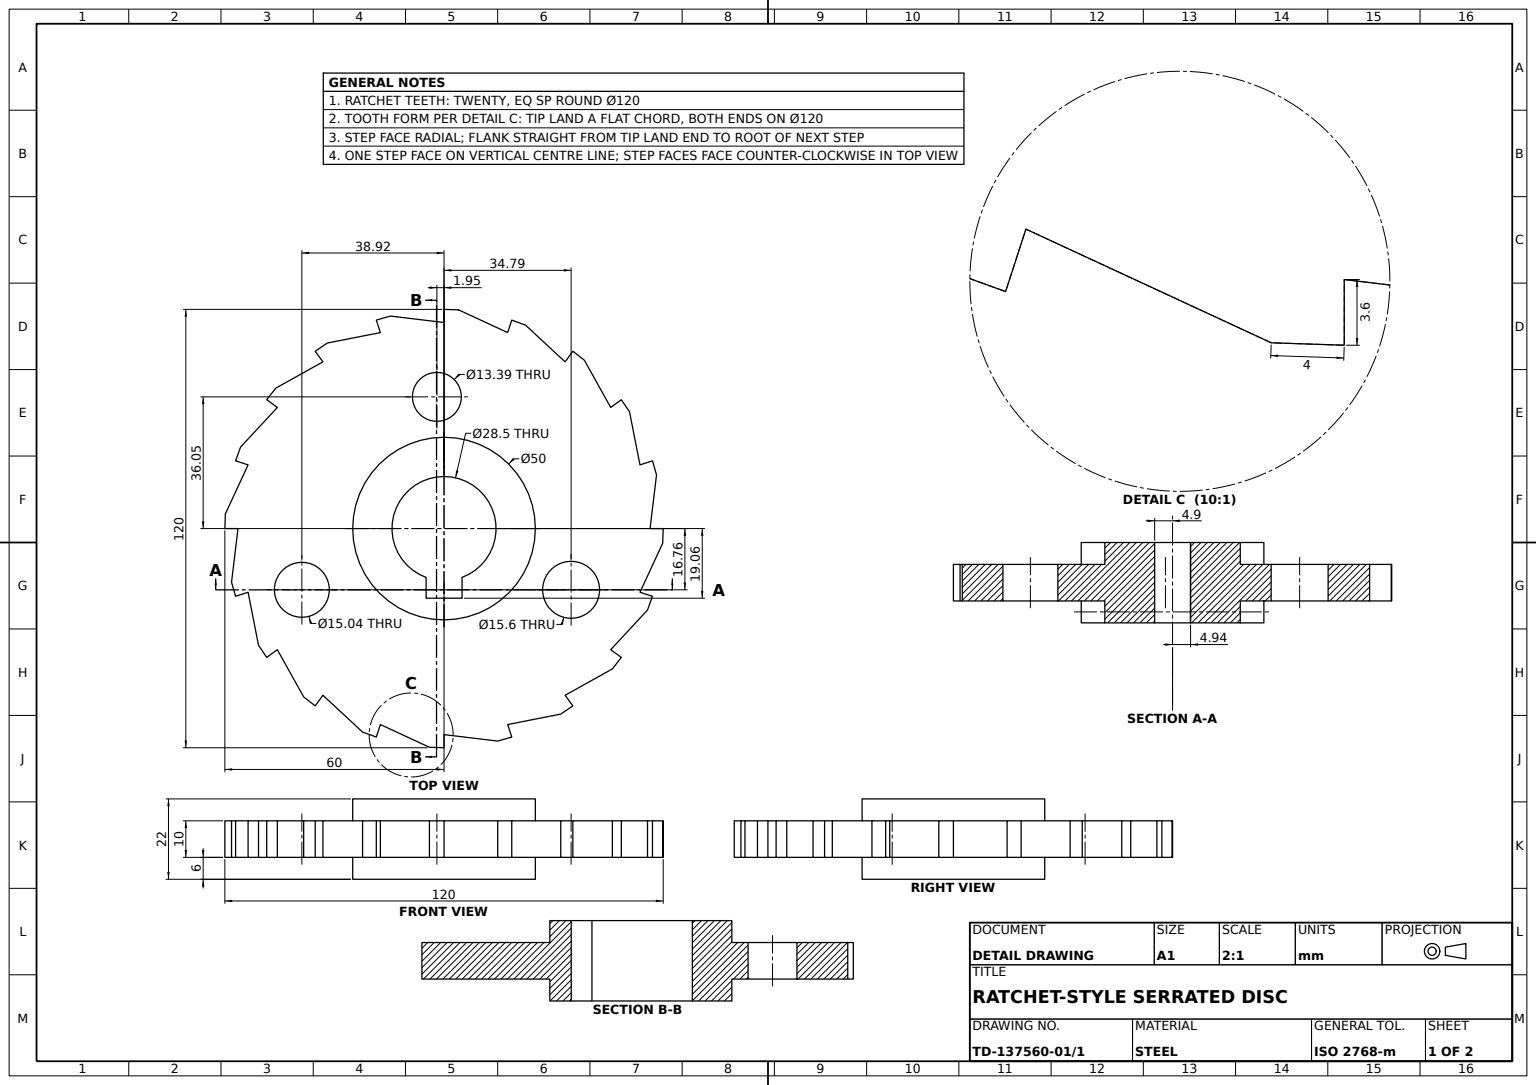
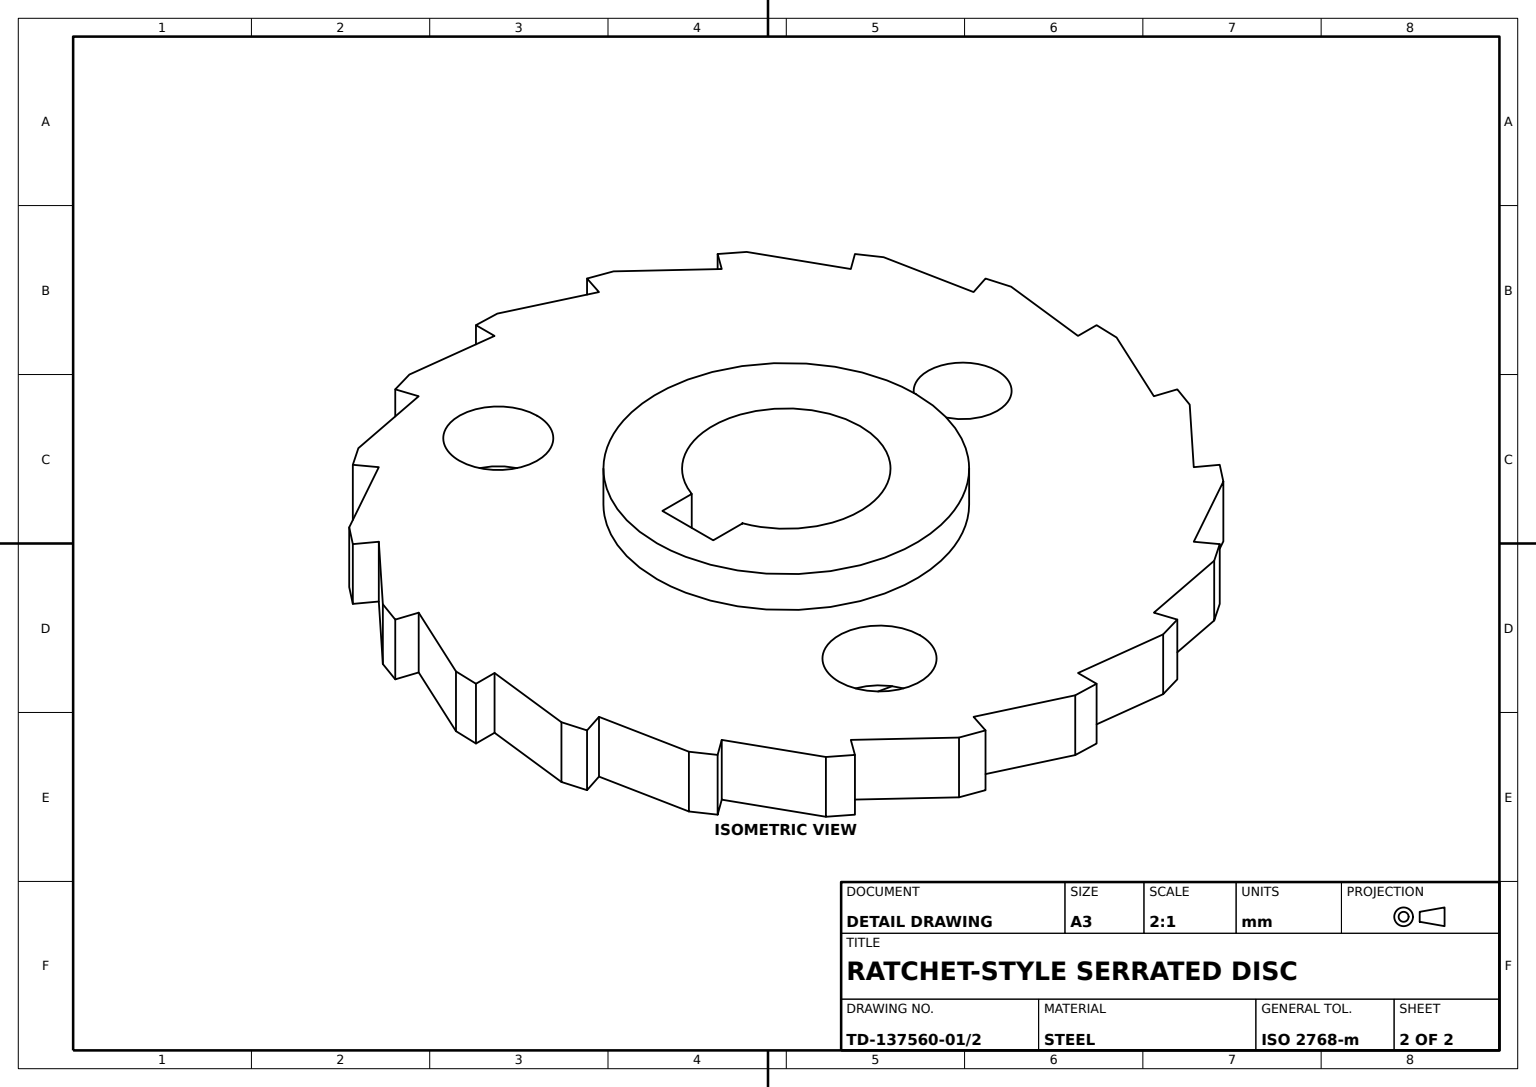
solid
v1 (59.866664,10,-3.997824)
v2 (59.866664,0,-3.997824)
e1 v1 v2 LINE
v3 (53.643191,0,-17.429729)
e2 v2 v3 LINE
v4 (53.643191,10,-17.429729)
e3 v4 v3 LINE
e4 v1 v4 LINE
face PLANE(AX(P(50.810937,10,-23.542486),D(-0.907338164,0,0.420401542),D(0.420401542,0,0.907338164))) rev [e1 e2 -e3 -e4]
v5 (0,10,60)
v6 (0,0,60)
e5 v5 v6 LINE
v7 (3.997824,0,59.866664)
e6 v6 v7 LINE
v8 (3.997824,10,59.866664)
e7 v8 v7 LINE
e8 v5 v8 LINE
face PLANE(AX(P(1.998912,10,59.933332),D(-0.033333726,0,-0.999444277),D(-0.999444277,0,0.033333726))) rev [e5 e6 -e7 -e8]
v9 (-57.063391,0,-18.54102)
v10 (-58.171976,0,-14.69766)
e9 v9 v10 LINE
v11 (-58.171976,10,-14.69766)
e10 v11 v10 LINE
v12 (-57.063391,10,-18.54102)
e11 v12 v11 LINE
e12 v12 v9 LINE
face PLANE(AX(P(-57.617684,10,-16.61934),D(0.96082868,0,0.277143009),D(0.277143009,0,-0.96082868))) rev [e9 -e10 -e11 e12]
v13 (-50.78301,0,-31.954434)
v14 (-53.643191,0,-17.429729)
e13 v13 v14 LINE
v15 (-53.643191,10,-17.429729)
e14 v15 v14 LINE
v16 (-50.78301,10,-31.954434)
e15 v16 v15 LINE
e16 v16 v13 LINE
face PLANE(AX(P(-54.944838,10,-10.819648),D(0.981157821,0,0.193208),D(0.193208,0,-0.981157821))) rev [e13 -e14 -e15 e16]
v17 (-35.267115,10,-48.54102)
v18 (-35.267115,0,-48.54102)
e17 v17 v18 LINE
v19 (-38.42305,0,-46.083286)
e18 v18 v19 LINE
v20 (-38.42305,10,-46.083286)
e19 v20 v19 LINE
e20 v17 v20 LINE
face PLANE(AX(P(-36.845082,10,-47.312153),D(0.614426157,0,0.788974333),D(0.788974333,0,-0.614426157))) rev [e17 e18 -e19 -e20]
v21 (-48.54102,10,35.267115)
v22 (-48.54102,0,35.267115)
e21 v21 v22 LINE
v23 (-45.631624,10,33.153316)
e22 v23 v21 LINE
v24 (-45.631624,0,33.153316)
e23 v23 v24 LINE
e24 v24 v22 LINE
face PLANE(AX(P(0,10,0),D(0.587785252,0,0.809016994),D(0.809016994,0,-0.587785252))) rev [-e21 -e22 e23 e24]
v25 (50.78301,10,31.954434)
v26 (50.78301,0,31.954434)
e25 v25 v26 LINE
v27 (48.54102,10,35.267115)
e26 v27 v25 LINE
v28 (48.54102,0,35.267115)
e27 v27 v28 LINE
e28 v28 v26 LINE
face PLANE(AX(P(49.662015,10,33.610775),D(-0.828160477,0,-0.560491056),D(-0.560491056,0,0.828160477))) rev [-e25 -e26 e27 e28]
v29 (58.171976,0,14.69766)
v30 (56.403789,0,0)
e29 v29 v30 LINE
v31 (56.403789,10,0)
e30 v31 v30 LINE
v32 (58.171976,10,14.69766)
e31 v32 v31 LINE
e32 v32 v29 LINE
face PLANE(AX(P(55.599101,10,-6.688792),D(-0.992841094,0,0.119442714),D(0.119442714,0,0.992841094))) rev [e29 -e30 -e31 e32]
v33 (55.701185,10,-22.301973)
v34 (45.631624,10,-33.153316)
e33 v33 v34 LINE
v35 (55.701185,0,-22.301973)
e34 v33 v35 LINE
v36 (45.631624,0,-33.153316)
e35 v35 v36 LINE
e36 v34 v36 LINE
face PLANE(AX(P(41.049045,10,-38.091678),D(-0.733018652,0,0.680208538),D(0.680208538,0,0.733018652))) rev [-e33 e34 e35 -e36]
v37 (-33.153316,10,-45.631624)
e37 v37 v17 LINE
v38 (-33.153316,0,-45.631624)
e38 v37 v38 LINE
e39 v38 v18 LINE
face PLANE(AX(P(0,10,0),D(-0.809016994,0,0.587785252),D(0.587785252,0,0.809016994))) rev [-e37 e38 e39 -e17]
v39 (18.54102,10,-57.063391)
v40 (18.54102,0,-57.063391)
e40 v39 v40 LINE
v41 (14.69766,0,-58.171976)
e41 v40 v41 LINE
v42 (14.69766,10,-58.171976)
e42 v42 v41 LINE
e43 v39 v42 LINE
face PLANE(AX(P(16.61934,10,-57.617684),D(-0.277143009,0,0.96082868),D(0.96082868,0,0.277143009))) rev [e40 e41 -e42 -e43]
v43 (-33.153316,10,45.631624)
v44 (-33.153316,0,45.631624)
e44 v43 v44 LINE
v45 (-35.267115,0,48.54102)
e45 v44 v45 LINE
v46 (-35.267115,10,48.54102)
e46 v46 v45 LINE
e47 v43 v46 LINE
face PLANE(AX(P(0,10,0),D(0.809016994,0,0.587785252),D(0.587785252,0,-0.809016994))) rev [e44 e45 -e46 -e47]
v47 (-59.866664,0,3.997824)
v48 (-53.643191,0,17.429729)
e48 v47 v48 LINE
v49 (-53.643191,10,17.429729)
e49 v49 v48 LINE
v50 (-59.866664,10,3.997824)
e50 v50 v49 LINE
e51 v50 v47 LINE
face PLANE(AX(P(-50.810937,10,23.542486),D(0.907338164,0,-0.420401542),D(-0.420401542,0,-0.907338164))) rev [e48 -e49 -e50 e51]
v51 (-4.898607,-6,-13.38156)
v52 (-4.898607,16,-13.38156)
e52 v51 v52 LINE
v53 (0,16,14.25)
e53 v52 v53 CIRCLE(AX(P(0,16,0),D(0,1,0),D(0,0,1)),14.25)
v54 (0,-6,14.25)
e54 v54 v53 LINE
e55 v51 v54 CIRCLE(AX(P(0,-6,0),D(0,1,0),D(0,0,1)),14.25)
face CYL(AX(P(0,-41,0),D(0,1,0),D(0,0,1)),14.25) rev [e52 e53 -e54 -e55]
v55 (57.063391,10,18.54102)
v56 (57.063391,0,18.54102)
e56 v55 v56 LINE
e57 v56 v29 LINE
e58 v55 v32 LINE
face PLANE(AX(P(57.617684,10,16.61934),D(-0.96082868,0,-0.277143009),D(-0.277143009,0,0.96082868))) rev [e56 e57 -e32 -e58]
v57 (0,16,25)
v58 (0,16,-25)
e59 v57 v58 CIRCLE(AX(P(0,16,0),D(0,1,0),D(0,0,1)),25)
e60 v58 v57 CIRCLE(AX(P(0,16,0),D(0,1,0),D(0,0,1)),25)
v59 (4.937063,16,-19.059359)
v60 (-4.898607,16,-19.059359)
e61 v59 v60 LINE
v61 (4.937063,16,-13.38156)
e62 v61 v59 LINE
v62 (4.898607,16,-13.38156)
e63 v62 v61 LINE
e64 v53 v62 CIRCLE(AX(P(0,16,0),D(0,1,0),D(0,0,1)),14.25)
e65 v60 v52 LINE
face PLANE(AX(P(0,16,0),D(0,1,0),D(0,0,1))) [e59 e60] [-e61 -e62 -e63 -e64 -e53 -e65]
v63 (-17.429729,10,-53.643191)
v64 (-17.429729,0,-53.643191)
e66 v63 v64 LINE
v65 (-18.54102,0,-57.063391)
e67 v64 v65 LINE
v66 (-18.54102,10,-57.063391)
e68 v66 v65 LINE
e69 v63 v66 LINE
face PLANE(AX(P(0,10,0),D(-0.951056516,0,0.309016994),D(0.309016994,0,0.951056516))) rev [e66 e67 -e68 -e69]
v67 (-17.429729,10,53.643191)
v68 (-17.429729,0,53.643191)
e70 v67 v68 LINE
v69 (-18.54102,0,57.063391)
e71 v68 v69 LINE
v70 (-18.54102,10,57.063391)
e72 v70 v69 LINE
e73 v67 v70 LINE
face PLANE(AX(P(0,10,0),D(0.951056516,0,0.309016994),D(0.309016994,0,-0.951056516))) rev [e70 e71 -e72 -e73]
v71 (17.429729,10,-53.643191)
e74 v71 v39 LINE
v72 (17.429729,0,-53.643191)
e75 v71 v72 LINE
e76 v72 v40 LINE
face PLANE(AX(P(0,10,0),D(-0.951056516,0,-0.309016994),D(-0.309016994,0,0.951056516))) rev [-e40 -e74 e75 e76]
v73 (48.54102,10,-35.267115)
e77 v34 v73 LINE
v74 (48.54102,0,-35.267115)
e78 v36 v74 LINE
e79 v73 v74 LINE
face PLANE(AX(P(0,10,0),D(-0.587785252,0,-0.809016994),D(-0.809016994,0,0.587785252))) rev [-e77 e36 e78 -e79]
v75 (-56.403789,10,0)
v76 (-56.403789,0,0)
e80 v75 v76 LINE
v77 (-60,0,0)
e81 v76 v77 LINE
v78 (-60,10,0)
e82 v78 v77 LINE
e83 v75 v78 LINE
face PLANE(AX(P(0,10,0),D(0,0,1),D(1,0,0))) rev [e80 e81 -e82 -e83]
v79 (-57.063391,0,18.54102)
e84 v48 v79 LINE
v80 (-57.063391,10,18.54102)
e85 v80 v79 LINE
e86 v49 v80 LINE
face PLANE(AX(P(0,10,0),D(0.309016994,0,0.951056516),D(0.951056516,0,-0.309016994))) rev [e49 e84 -e85 -e86]
v81 (33.153316,0,-45.631624)
v82 (35.267115,0,-48.54102)
e87 v81 v82 LINE
v83 (35.267115,10,-48.54102)
e88 v83 v82 LINE
v84 (33.153316,10,-45.631624)
e89 v84 v83 LINE
e90 v84 v81 LINE
face PLANE(AX(P(0,10,0),D(-0.809016994,0,-0.587785252),D(-0.587785252,0,0.809016994))) rev [e87 -e88 -e89 e90]
v85 (0,-6,25)
v86 (0,0,25)
e91 v85 v86 LINE
v87 (0,-6,-25)
e92 v85 v87 CIRCLE(AX(P(0,-6,0),D(0,1,0),D(0,0,1)),25)
v88 (0,0,-25)
e93 v87 v88 LINE
e94 v86 v88 CIRCLE(AX(P(0,0,0),D(0,1,0),D(0,0,1)),25)
face CYL(AX(P(0,-6,0),D(0,1,0),D(0,0,1)),25) [-e91 e92 e93 -e94]
v89 (18.54102,0,57.063391)
v90 (22.301973,0,55.701185)
e95 v89 v90 LINE
v91 (22.301973,10,55.701185)
e96 v91 v90 LINE
v92 (18.54102,10,57.063391)
e97 v92 v91 LINE
e98 v92 v89 LINE
face PLANE(AX(P(20.421496,10,56.382288),D(-0.340547524,0,-0.940227305),D(-0.940227305,0,0.340547524))) rev [e95 -e96 -e97 e98]
v93 (-3.997824,10,-59.866664)
e99 v93 v63 LINE
v94 (-3.997824,0,-59.866664)
e100 v93 v94 LINE
e101 v94 v64 LINE
face PLANE(AX(P(-23.542486,10,-50.810937),D(0.420401542,0,0.907338164),D(0.907338164,0,-0.420401542))) rev [-e99 e100 e101 -e66]
e102 v10 v76 LINE
e103 v14 v9 LINE
v95 (-48.54102,0,-35.267115)
e104 v95 v13 LINE
v96 (-45.631624,0,-33.153316)
e105 v96 v95 LINE
e106 v19 v96 LINE
v97 (-22.301973,0,-55.701185)
e107 v97 v38 LINE
e108 v65 v97 LINE
v98 (0,0,-60)
e109 v98 v94 LINE
v99 (0,0,-56.403789)
e110 v99 v98 LINE
e111 v41 v99 LINE
v100 (31.954434,0,-50.78301)
e112 v100 v72 LINE
e113 v82 v100 LINE
v101 (46.083286,0,-38.42305)
e114 v101 v81 LINE
e115 v74 v101 LINE
v102 (57.063391,0,-18.54102)
e116 v102 v35 LINE
e117 v3 v102 LINE
v103 (60,0,0)
e118 v103 v2 LINE
e119 v30 v103 LINE
v104 (53.643191,0,17.429729)
e120 v104 v56 LINE
e121 v26 v104 LINE
v105 (45.631624,0,33.153316)
e122 v105 v28 LINE
v106 (38.42305,0,46.083286)
e123 v106 v105 LINE
v107 (35.267115,0,48.54102)
e124 v107 v106 LINE
v108 (33.153316,0,45.631624)
e125 v108 v107 LINE
e126 v90 v108 LINE
v109 (17.429729,0,53.643191)
e127 v109 v89 LINE
e128 v7 v109 LINE
v110 (0,0,56.403789)
e129 v110 v6 LINE
v111 (-14.69766,0,58.171976)
e130 v111 v110 LINE
e131 v69 v111 LINE
v112 (-31.954434,0,50.78301)
e132 v112 v68 LINE
e133 v45 v112 LINE
v113 (-46.083286,0,38.42305)
e134 v113 v44 LINE
e135 v22 v113 LINE
v114 (-55.701185,0,22.301973)
e136 v114 v24 LINE
e137 v79 v114 LINE
e138 v77 v47 LINE
v115 (34.789071,0,-24.563742)
v116 (34.789071,0,-8.962359)
e139 v115 v116 CIRCLE(AX(P(34.789071,0,-16.763051),D(0,-1,0),D(0,0,1)),7.800692)
e140 v116 v115 CIRCLE(AX(P(34.789071,0,-16.763051),D(0,-1,0),D(0,0,1)),7.800692)
v117 (-38.922426,0,-24.284994)
v118 (-38.922426,0,-9.241107)
e141 v117 v118 CIRCLE(AX(P(-38.922426,0,-16.763051),D(0,-1,0),D(0,0,1)),7.521943)
e142 v118 v117 CIRCLE(AX(P(-38.922426,0,-16.763051),D(0,-1,0),D(0,0,1)),7.521943)
e143 v88 v86 CIRCLE(AX(P(0,0,0),D(0,1,0),D(0,0,1)),25)
v119 (-1.951862,0,42.746873)
v120 (-1.951862,0,29.357209)
e144 v119 v120 CIRCLE(AX(P(-1.951862,0,36.052041),D(0,-1,0),D(0,0,1)),6.694832)
e145 v120 v119 CIRCLE(AX(P(-1.951862,0,36.052041),D(0,-1,0),D(0,0,1)),6.694832)
face PLANE(AX(P(0,0,0),D(0,1,0),D(0,0,1))) rev [-e102 -e9 -e103 -e13 -e104 -e105 -e106 -e18 -e39 -e107 -e108 -e67 -e101 -e109 -e110 -e111 -e41 -e76 -e112 -e113 -e87 -e114 -e115 -e78 -e35 -e116 -e117 -e2 -e118 -e119 -e29 -e57 -e120 -e121 -e28 -e122 -e123 -e124 -e125 -e126 -e95 -e127 -e128 -e6 -e129 -e130 -e131 -e71 -e132 -e133 -e45 -e134 -e135 -e24 -e136 -e137 -e84 -e48 -e138 -e81] [-e139 -e140] [-e141 -e142] [e94 e143] [-e144 -e145]
e146 v87 v85 CIRCLE(AX(P(0,-6,0),D(0,1,0),D(0,0,1)),25)
face CYL(AX(P(0,-6,0),D(0,1,0),D(0,0,1)),25) [-e143 -e93 e146 e91]
v121 (0,10,56.403789)
e147 v121 v110 LINE
v122 (-14.69766,10,58.171976)
e148 v122 v121 LINE
e149 v122 v111 LINE
face PLANE(AX(P(6.688792,10,55.599101),D(-0.119442714,0,-0.992841094),D(-0.992841094,0,0.119442714))) rev [e130 -e147 -e148 e149]
v123 (-46.083286,10,38.42305)
e150 v123 v113 LINE
e151 v21 v123 LINE
face PLANE(AX(P(-47.312153,10,36.845082),D(0.788974333,0,-0.614426157),D(-0.614426157,0,-0.788974333))) rev [-e150 -e151 e21 e135]
v124 (0,10,-56.403789)
e152 v42 v124 LINE
e153 v124 v99 LINE
face PLANE(AX(P(-6.688792,10,-55.599101),D(0.119442714,0,0.992841094),D(0.992841094,0,-0.119442714))) rev [-e152 e42 e111 -e153]
v125 (57.063391,10,-18.54102)
e154 v125 v33 LINE
e155 v125 v102 LINE
face PLANE(AX(P(56.382288,10,-20.421496),D(-0.940227305,0,0.340547524),D(0.340547524,0,0.940227305))) rev [-e154 e155 e116 -e34]
v126 (60,10,0)
e156 v126 v1 LINE
e157 v126 v103 LINE
face PLANE(AX(P(59.933332,10,-1.998912),D(-0.999444277,0,0.033333726),D(0.033333726,0,0.999444277))) rev [e118 -e1 -e156 e157]
v127 (31.954434,10,-50.78301)
e158 v127 v71 LINE
e159 v127 v100 LINE
face PLANE(AX(P(10.819648,10,-54.944838),D(-0.193208,0,0.981157821),D(0.981157821,0,0.193208))) rev [-e75 -e158 e159 e112]
v128 (34.789071,10,-24.563742)
v129 (34.789071,10,-8.962359)
e160 v128 v129 CIRCLE(AX(P(34.789071,10,-16.763051),D(0,-1,0),D(0,0,1)),7.800692)
e161 v128 v115 LINE
e162 v129 v116 LINE
face CYL(AX(P(34.789071,57,-16.763051),D(0,-1,0),D(0,0,-1)),7.800692) rev [-e160 e161 e139 -e162]
v130 (-55.701185,10,22.301973)
e163 v130 v23 LINE
e164 v130 v114 LINE
face PLANE(AX(P(-41.049045,10,38.091678),D(0.733018652,0,-0.680208538),D(-0.680208538,0,-0.733018652))) rev [e136 -e23 -e163 e164]
v131 (-1.951862,10,42.746873)
e165 v131 v119 LINE
v132 (-1.951862,10,29.357209)
e166 v132 v131 CIRCLE(AX(P(-1.951862,10,36.052041),D(0,-1,0),D(0,0,1)),6.694832)
e167 v132 v120 LINE
face CYL(AX(P(-1.951862,57,36.052041),D(0,-1,0),D(0,0,-1)),6.694832) rev [-e165 -e166 e167 e145]
v133 (46.083286,10,-38.42305)
e168 v133 v84 LINE
e169 v133 v101 LINE
face PLANE(AX(P(27.268985,10,-48.912191),D(-0.486946168,0,0.873431983),D(0.873431983,0,0.486946168))) rev [-e168 e169 e114 -e90]
e170 v11 v75 LINE
face PLANE(AX(P(-55.599101,10,6.688792),D(0.992841094,0,-0.119442714),D(-0.119442714,0,-0.992841094))) rev [e102 -e80 -e170 e10]
v134 (45.631624,10,33.153316)
e171 v134 v27 LINE
e172 v134 v105 LINE
face PLANE(AX(P(0,10,0),D(0.587785252,0,-0.809016994),D(-0.809016994,0,-0.587785252))) rev [-e27 -e171 e172 e122]
v135 (4.937063,-6,-13.38156)
v136 (4.937063,-6,-19.059359)
e173 v135 v136 LINE
e174 v135 v61 LINE
e175 v136 v59 LINE
face PLANE(AX(P(4.937063,-41,-13.38156),D(1,0,0),D(0,0,-1))) rev [-e173 e174 e62 -e175]
e176 v123 v43 LINE
face PLANE(AX(P(-27.268985,10,48.912191),D(0.486946168,0,-0.873431983),D(-0.873431983,0,-0.486946168))) rev [e150 e134 -e44 -e176]
v137 (53.643191,10,17.429729)
e177 v137 v104 LINE
e178 v25 v137 LINE
face PLANE(AX(P(54.944838,10,10.819648),D(-0.981157821,0,-0.193208),D(-0.193208,0,0.981157821))) rev [e121 -e177 -e178 e25]
v138 (-22.301973,10,-55.701185)
e179 v138 v97 LINE
e180 v138 v37 LINE
face PLANE(AX(P(-38.091678,10,-41.049045),D(0.680208538,0,0.733018652),D(0.733018652,0,-0.680208538))) rev [e179 e107 -e38 -e180]
v139 (38.42305,10,46.083286)
e181 v139 v106 LINE
e182 v139 v134 LINE
face PLANE(AX(P(48.912191,10,27.268985),D(-0.873431983,0,-0.486946168),D(-0.486946168,0,0.873431983))) rev [e181 e123 -e172 -e182]
v140 (-38.922426,10,-24.284994)
e183 v140 v117 LINE
v141 (-38.922426,10,-9.241107)
e184 v141 v118 LINE
e185 v140 v141 CIRCLE(AX(P(-38.922426,10,-16.763051),D(0,-1,0),D(0,0,1)),7.521943)
face CYL(AX(P(-38.922426,57,-16.763051),D(0,-1,0),D(0,0,-1)),7.521943) rev [e183 e141 -e184 -e185]
e186 v15 v12 LINE
face PLANE(AX(P(0,10,0),D(-0.309016994,0,0.951056516),D(0.951056516,0,0.309016994))) rev [e103 -e12 -e186 e14]
v142 (-48.54102,10,-35.267115)
e187 v142 v95 LINE
e188 v142 v16 LINE
face PLANE(AX(P(-49.662015,10,-33.610775),D(0.828160477,0,0.560491056),D(0.560491056,0,-0.828160477))) rev [e187 e104 -e16 -e188]
e189 v131 v132 CIRCLE(AX(P(-1.951862,10,36.052041),D(0,-1,0),D(0,0,1)),6.694832)
face CYL(AX(P(-1.951862,57,36.052041),D(0,-1,0),D(0,0,-1)),6.694832) rev [-e167 -e189 e165 e144]
e190 v80 v130 LINE
face PLANE(AX(P(-56.382288,10,20.421496),D(0.940227305,0,-0.340547524),D(-0.340547524,0,-0.940227305))) rev [-e190 e85 e137 -e164]
e191 v31 v126 LINE
face PLANE(AX(P(0,10,0),D(0,0,-1),D(-1,0,0))) rev [-e191 e30 e119 -e157]
e192 v129 v128 CIRCLE(AX(P(34.789071,10,-16.763051),D(0,-1,0),D(0,0,1)),7.800692)
face CYL(AX(P(34.789071,57,-16.763051),D(0,-1,0),D(0,0,-1)),7.800692) rev [-e192 e162 e140 -e161]
v143 (33.153316,10,45.631624)
e193 v91 v143 LINE
e194 v143 v108 LINE
face PLANE(AX(P(38.091678,10,41.049045),D(-0.680208538,0,-0.733018652),D(-0.733018652,0,0.680208538))) rev [-e193 e96 e126 -e194]
v144 (-4.898607,-6,-19.059359)
e195 v144 v51 LINE
v145 (4.898607,-6,-13.38156)
e196 v54 v145 CIRCLE(AX(P(0,-6,0),D(0,1,0),D(0,0,1)),14.25)
e197 v145 v135 LINE
e198 v136 v144 LINE
face PLANE(AX(P(0,-6,0),D(0,1,0),D(0,0,1))) rev [e195 e55 e196 e197 e173 e198] [-e92 -e146]
v146 (0,10,-60)
e199 v146 v93 LINE
e200 v146 v98 LINE
face PLANE(AX(P(-1.998912,10,-59.933332),D(0.033333726,0,0.999444277),D(0.999444277,0,-0.033333726))) rev [e109 -e100 -e199 e200]
v147 (-45.631624,10,-33.153316)
e201 v147 v96 LINE
e202 v20 v147 LINE
face PLANE(AX(P(-48.912191,10,-27.268985),D(0.873431983,0,0.486946168),D(0.486946168,0,-0.873431983))) rev [e19 e106 -e201 -e202]
e203 v141 v140 CIRCLE(AX(P(-38.922426,10,-16.763051),D(0,-1,0),D(0,0,1)),7.521943)
face CYL(AX(P(-38.922426,57,-16.763051),D(0,-1,0),D(0,0,-1)),7.521943) rev [e184 e142 -e183 -e203]
v148 (0,10,-25)
e204 v148 v58 LINE
v149 (0,10,25)
e205 v148 v149 CIRCLE(AX(P(0,10,0),D(0,1,0),D(0,0,1)),25)
e206 v149 v57 LINE
face CYL(AX(P(0,-6,0),D(0,1,0),D(0,0,1)),25) [-e60 -e204 e205 e206]
e207 v121 v5 LINE
face PLANE(AX(P(0,10,0),D(1,0,0),D(0,0,-1))) rev [-e5 -e207 e147 e129]
e208 v83 v127 LINE
face PLANE(AX(P(33.610775,10,-49.662015),D(-0.560491056,0,0.828160477),D(0.828160477,0,0.560491056))) rev [-e159 -e208 e88 e113]
e209 v149 v148 CIRCLE(AX(P(0,10,0),D(0,1,0),D(0,0,1)),25)
v150 (-31.954434,10,50.78301)
e210 v46 v150 LINE
e211 v150 v67 LINE
e212 v70 v122 LINE
v151 (17.429729,10,53.643191)
e213 v8 v151 LINE
e214 v151 v92 LINE
v152 (35.267115,10,48.54102)
e215 v143 v152 LINE
e216 v152 v139 LINE
e217 v137 v55 LINE
e218 v4 v125 LINE
e219 v73 v133 LINE
e220 v124 v146 LINE
e221 v66 v138 LINE
e222 v147 v142 LINE
e223 v78 v50 LINE
face PLANE(AX(P(0,10,0),D(0,1,0),D(0,0,1))) [-e209 -e205] [e151 e176 e47 e210 e211 e73 e212 e148 e207 e8 e213 e214 e97 e193 e215 e216 e182 e171 e26 e178 e217 e58 e31 e191 e156 e4 e218 e154 e33 e77 e219 e168 e89 e208 e158 e74 e43 e152 e220 e199 e99 e69 e221 e180 e37 e20 e202 e222 e188 e15 e186 e11 e170 e83 e223 e50 e86 e190 e163 e22] [e160 e192] [e166 e189] [e185 e203]
face PLANE(AX(P(0,10,0),D(-0.587785252,0,0.809016994),D(0.809016994,0,0.587785252))) rev [-e222 e201 e105 -e187]
face PLANE(AX(P(-20.421496,10,-56.382288),D(0.340547524,0,0.940227305),D(0.940227305,0,-0.340547524))) rev [-e221 e68 e108 -e179]
face PLANE(AX(P(0,10,0),D(0.309016994,0,-0.951056516),D(-0.951056516,0,-0.309016994))) rev [e120 -e56 -e217 e177]
e224 v151 v109 LINE
face PLANE(AX(P(0,10,0),D(0.951056516,0,-0.309016994),D(-0.309016994,0,-0.951056516))) rev [-e214 e224 e127 -e98]
e225 v152 v107 LINE
face PLANE(AX(P(36.845082,10,47.312153),D(-0.614426157,0,-0.788974333),D(-0.788974333,0,0.614426157))) rev [e124 -e181 -e216 e225]
face PLANE(AX(P(47.312153,10,-36.845082),D(-0.788974333,0,0.614426157),D(0.614426157,0,0.788974333))) rev [e79 e115 -e169 -e219]
face PLANE(AX(P(-59.933332,10,1.998912),D(0.999444277,0,-0.033333726),D(-0.033333726,0,-0.999444277))) rev [e82 e138 -e51 -e223]
e226 v145 v62 LINE
face PLANE(AX(P(4.898607,-41,-13.38156),D(0,0,1),D(1,0,0))) rev [-e174 -e197 e226 e63]
face PLANE(AX(P(-16.61934,10,57.617684),D(0.277143009,0,-0.96082868),D(-0.96082868,0,-0.277143009))) rev [e131 -e149 -e212 e72]
face PLANE(AX(P(0,10,0),D(-1,0,0),D(0,0,1))) rev [e153 e110 -e200 -e220]
face PLANE(AX(P(23.542486,10,50.810937),D(-0.420401542,0,-0.907338164),D(-0.907338164,0,0.420401542))) rev [-e224 -e213 e7 e128]
face PLANE(AX(P(0,10,0),D(-0.309016994,0,-0.951056516),D(-0.951056516,0,0.309016994))) rev [e117 -e155 -e218 e3]
e227 v150 v112 LINE
face PLANE(AX(P(-33.610775,10,49.662015),D(0.560491056,0,-0.828160477),D(-0.828160477,0,-0.560491056))) rev [-e227 -e210 e46 e133]
face CYL(AX(P(0,-6,0),D(0,1,0),D(0,0,1)),25) [e209 e204 -e59 -e206]
face PLANE(AX(P(0,10,0),D(0.809016994,0,-0.587785252),D(-0.587785252,0,-0.809016994))) rev [e125 -e225 -e215 e194]
e228 v144 v60 LINE
face PLANE(AX(P(-4.898607,-41,-19.059359),D(0,0,-1),D(-1,0,0))) rev [-e228 -e198 e175 e61]
face PLANE(AX(P(-4.898607,-41,-13.38156),D(-1,0,0),D(0,0,1))) rev [e65 -e52 -e195 e228]
face CYL(AX(P(0,-41,0),D(0,1,0),D(0,0,1)),14.25) rev [e64 -e226 -e196 e54]
face PLANE(AX(P(-10.819648,10,54.944838),D(0.193208,0,-0.981157821),D(-0.981157821,0,-0.193208))) rev [-e70 -e211 e227 e132]
